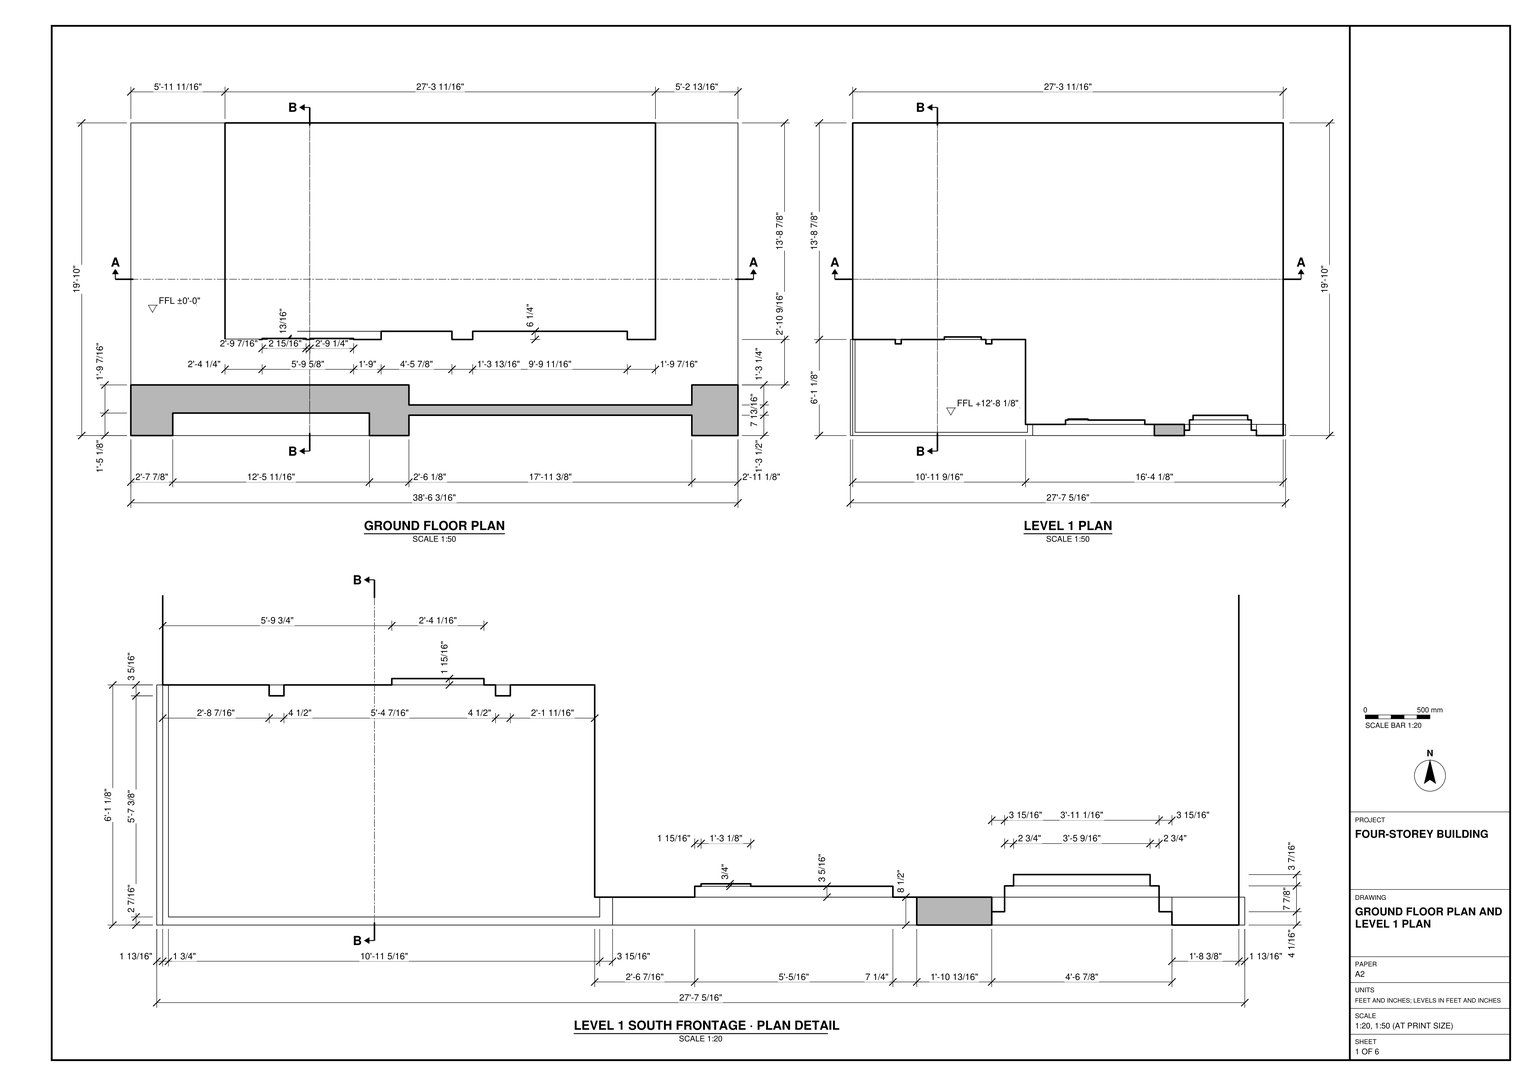
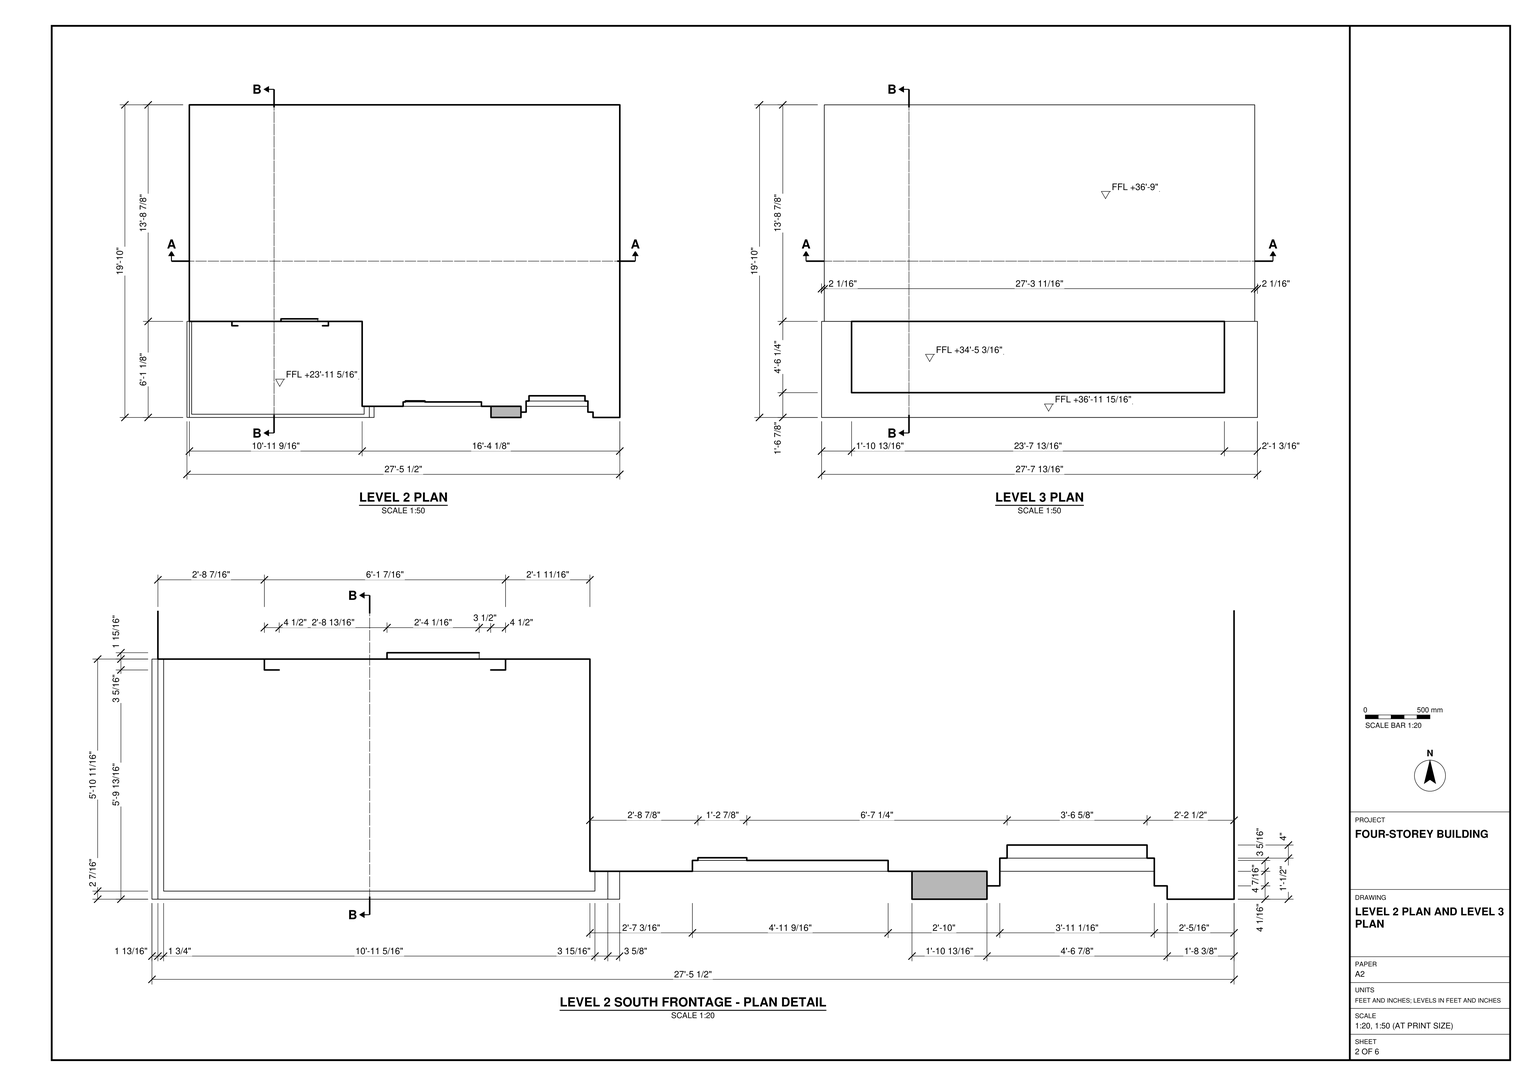
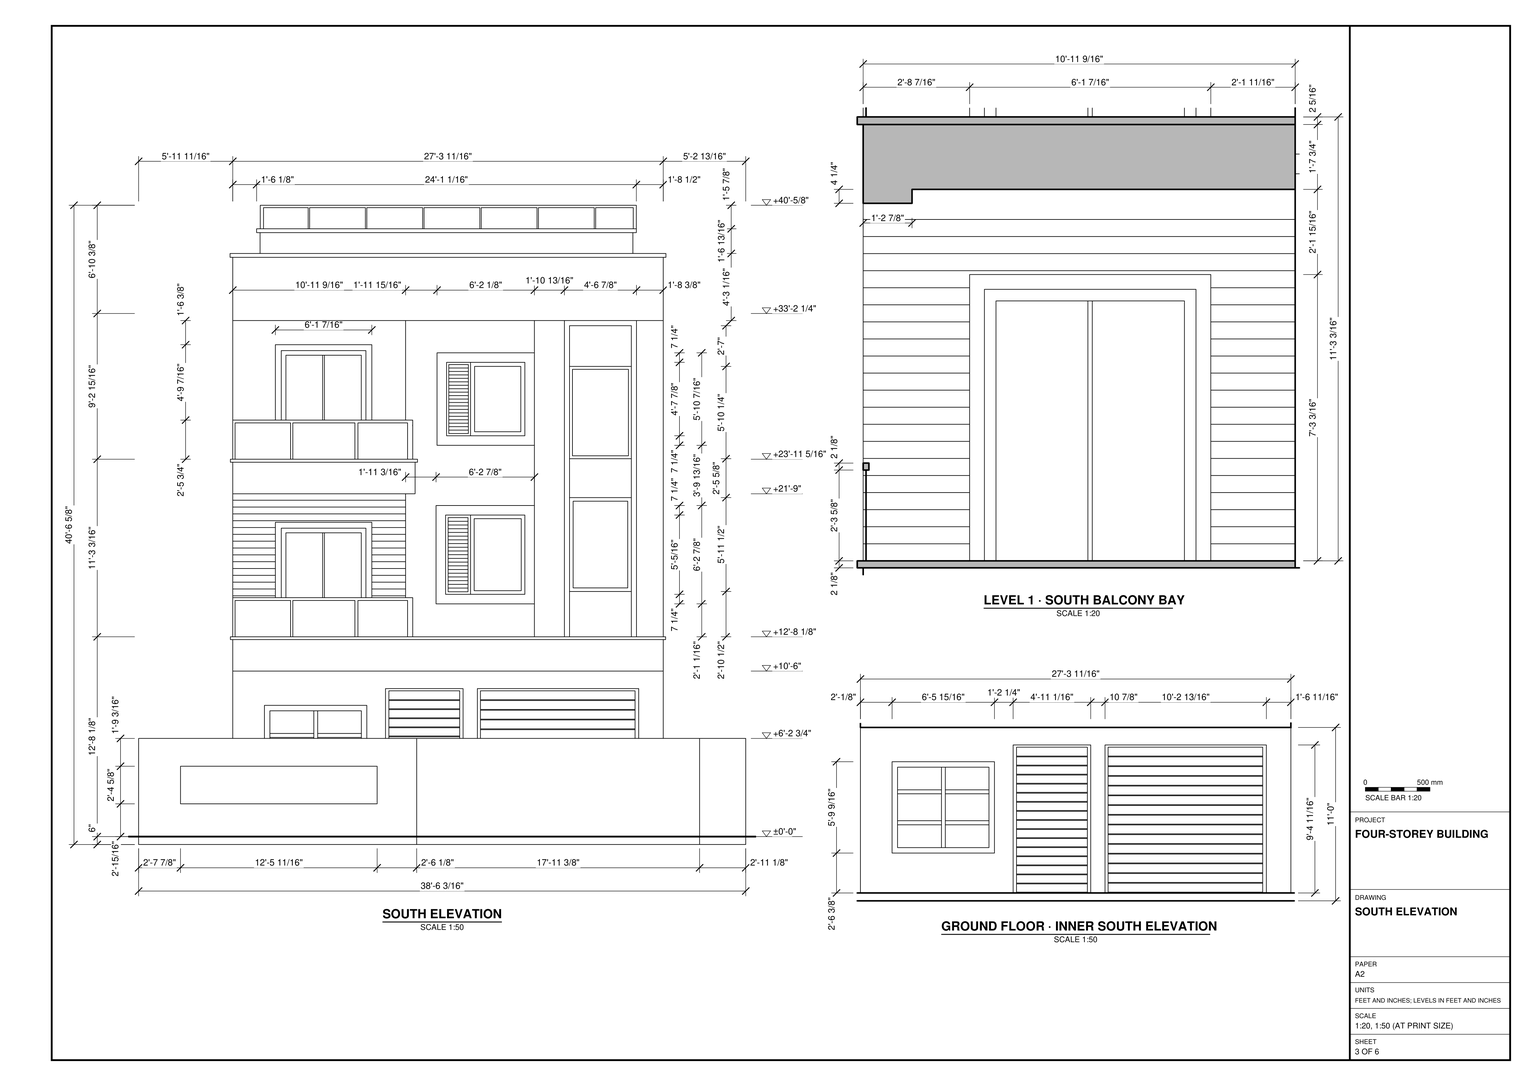
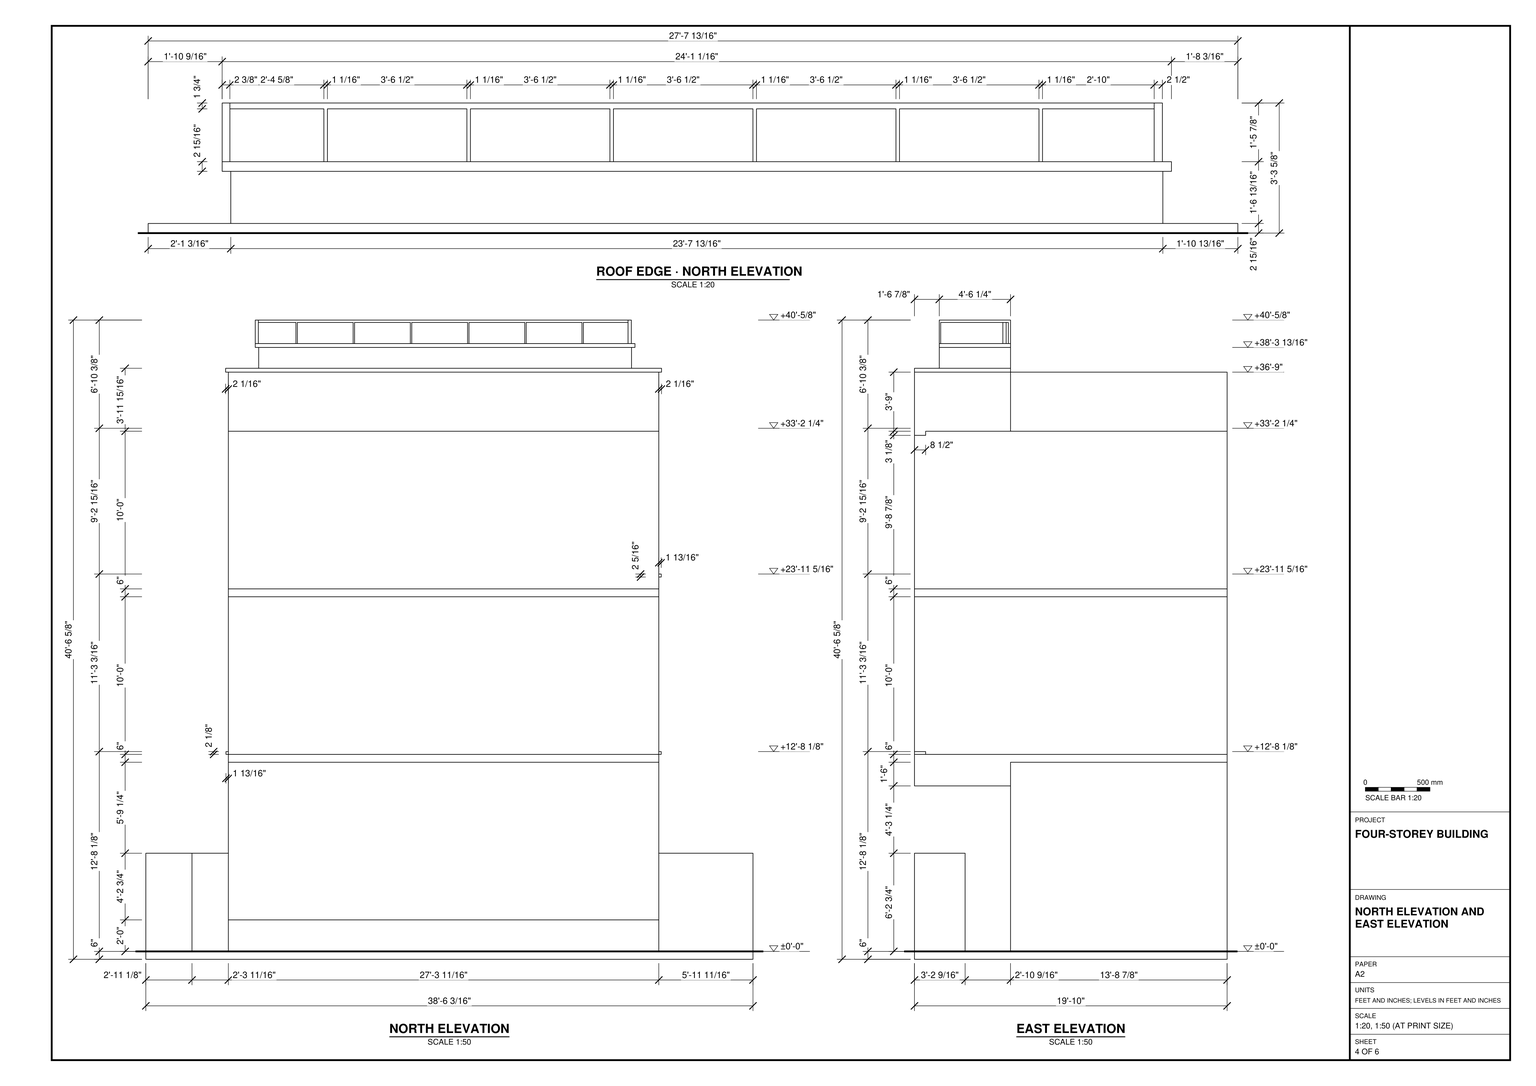
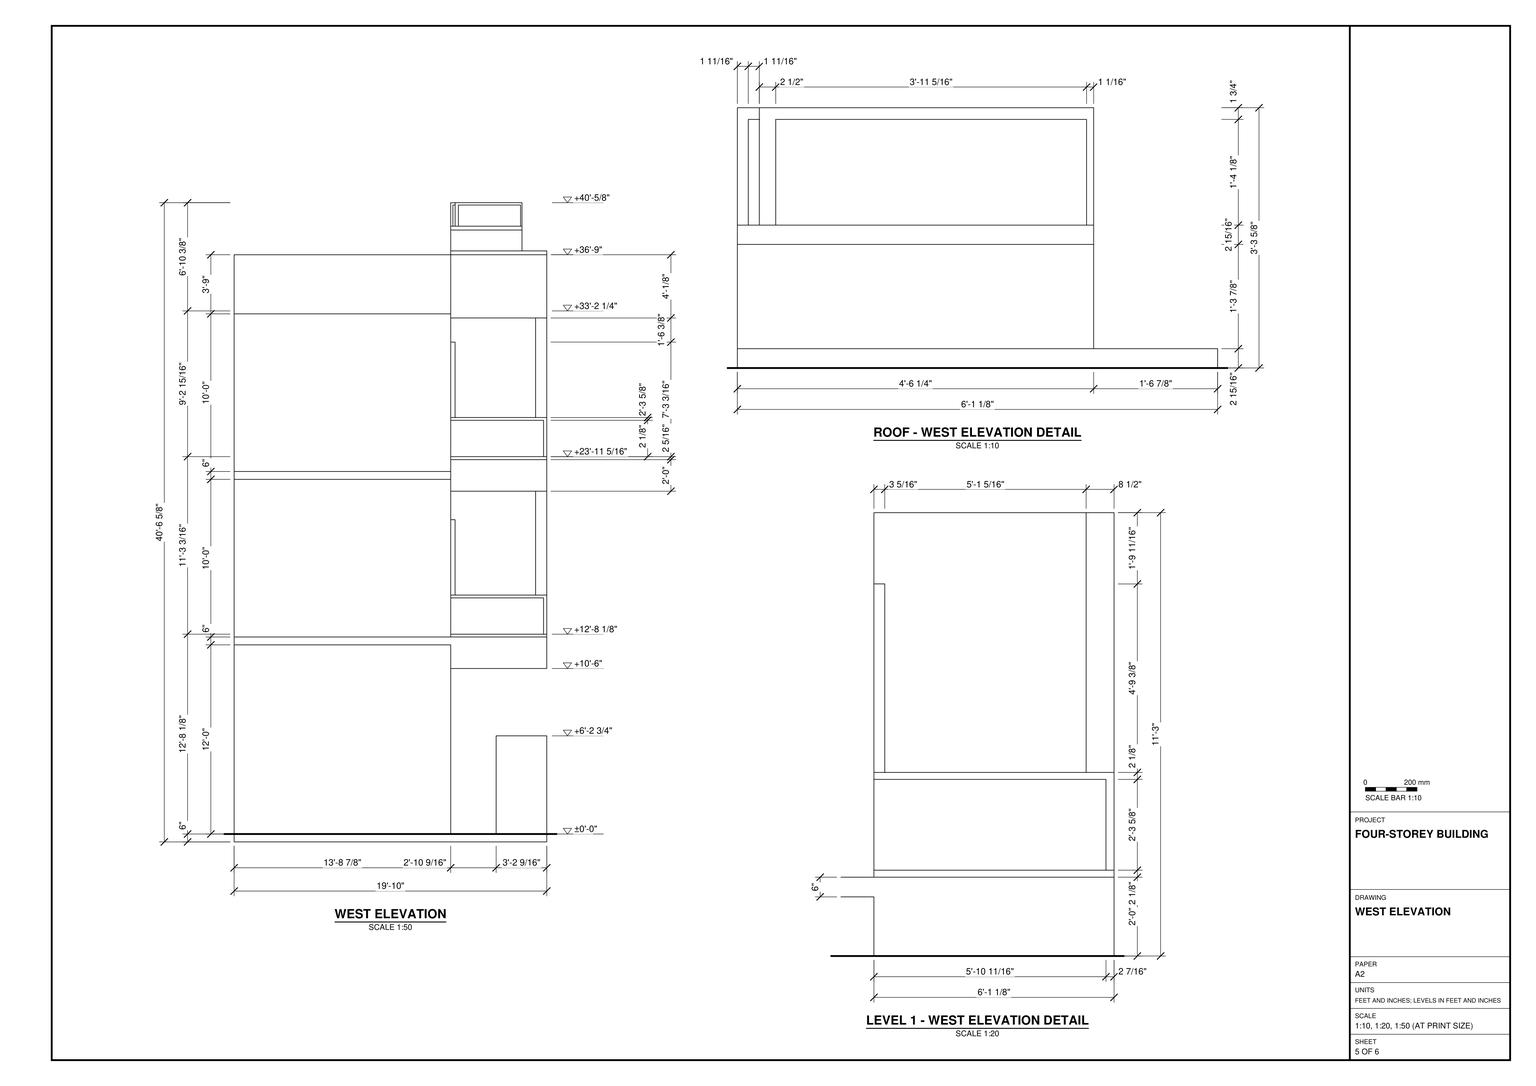
Build the four-storey building in SketchUp from task_files/diagram_01.pdf. Work in feet and inches. Set the overall width to 38'-6 3/16", depth to 19'-10" and height to 40'-6 5/8". Use ±0'-0" for the ground floor and +12'-8 1/8", +23'-11 5/16" and +33'-2 1/4" for the successive levels.

Set out the south frontage wall separately from the narrower building behind it. Match the wall thicknesses, setbacks and changes in profile to the plans. On the inner ground-floor elevation, place the divided window on the left and the narrow and wide horizontally slatted openings to its right. Model the floor slabs and stack the balconies on the left of the south elevation. Show their projecting slab edges, panelled guards and recessed paired doors. Use the enlarged balcony view for the horizontal courses around the lower balcony doors. To the right of the balconies, distinguish the windows with louvred side panels from the tall framed bay. Finish the roof with the changes in height shown in the level 3 plan and south elevation.

Keep shell elements such as walls, slabs and roof in separate groups or components. Keep each furniture or joinery piece shown separate and use components for repeated parts. Any decor or loose items shown may use suitable library components. Save one SketchUp model as output_files/four_storey_building_with_stacked_south_balconies.skp.

# SketchUp Ruby script. Lengths in inches.
U = 1.inch
M = Sketchup.active_model
def pt(a) = Geom::Point3d.new(a.map { |v| v * U })
def face(e, loops, mat)
  f = e.add_face(loops[0].map { |a| pt(a) })
  loops[1..].each { |l| e.add_face(l.map { |a| pt(a) }).erase! }
  f.material = f.back_material = mat if mat
  f
end
# faces: each face lists its corners as indices into pts; further lists are holes
def faces(e, pts, list, mat = nil) = list.each { |f| face(e, (f[0].is_a?(Array) ? f : [f]).map { |l| l.map { |i| pts[i] } }, mat) }
# xy, xz, yz: faces in a plane at the given z, y or x. An outline is a flat list of corners, or four numbers for a rectangle; further outlines are holes
def ring(l) = l.size == 4 ? [[l[0], l[1]], [l[2], l[1]], [l[2], l[3]], [l[0], l[3]]] : l.each_slice(2).to_a
def flat(e, list, mat, &to3) = list.each { |f| face(e, (f[0].is_a?(Array) ? f : [f]).map { |l| ring(l).map { |u, v| to3.(u, v) } }, mat) }
def xy(e, z, list, mat = nil) = flat(e, list, mat) { |x, y| [x, y, z] }
def xz(e, y, list, mat = nil) = flat(e, list, mat) { |x, z| [x, y, z] }
def yz(e, x, list, mat = nil) = flat(e, list, mat) { |y, z| [x, y, z] }
def lines(e, pts, list) = list.each { |a, b| e.add_line(pt(pts[a]), pt(pts[b])) }
# prism: a flat outline (further loops are holes) pulled along v
def prism(e, loops, v, mat = nil)
  f = face(e, loops, mat); d = Geom::Vector3d.new(v.map { |x| x * U })
  f.pushpull(f.normal.samedirection?(d) ? d.length : -d.length)
end
def box(e, o, s, mat = nil) = prism(e, [[o, [o[0] + s[0], o[1], o[2]], [o[0] + s[0], o[1] + s[1], o[2]], [o[0], o[1] + s[1], o[2]]]], [0, 0, s[2]], mat)
def at(x, y, z, deg = 0) = Geom::Transformation.translation(pt([x, y, z])) * Geom::Transformation.rotation(ORIGIN, Z_AXIS, deg.degrees)
def axes(o, x, y, z) = Geom::Transformation.new([*x, 0, *y, 0, *z, 0, *pt(o).to_a, 1])
def part(name) = M.definitions.add(name)
# library, detail: a bought-in or finely detailed component or shape, given as its bounding box
def library(name, o, s) = part(name).tap { |d| box(d.entities, o, s) }
def detail(e, o, s) = box(e.add_group.entities, o, s)
def put(e, d, t, mat = nil) = e.add_instance(d, t).tap { |i| i.material = mat if mat }
def group(e, t, mat = nil) = e.add_group.tap { |g| g.transformation = t; g.material = mat if mat }.entities
root = M.entities
M.materials.add("[0009_Linen]").color = [250, 240, 230]
M.materials.add("[0137_Black]").color = [0, 0, 0]
M.materials.add("[Translucent Glass Gray]").color = [252, 252, 252]
M.materials["[Translucent Glass Gray]"].alpha = 0.5
M.materials.add("[Wood Bamboo]").color = [177, 105, 43]
M.materials.add("[Wood Fence with Lattice]").color = [170, 106, 61]
xy(root,-24,[[0,0,0,238,462.1875,238,462.1875,0,427.0625,0,427.0625,15.5,211.7,15.5,211.7,0]])
xy(root,-18,[[211.7,23.29,427.0625,23.29,427.0625,38.54,462.1875,38.54,462.1875,238,399.375,238,399.375,73.125,377.92,73.125,377.92,79.375,260.24,79.375,260.24,73.125,244.4375,73.125,244.4375,79.375,190.53,79.375,190.53,73.125,71.6875,73.125,71.6875,238,0,238,0,38.54,211.7,38.54]])
xy(root,6.95,[[31.9,0,181.59,17.125]])
xy(root,16.52,[[99.95,73.125,133.38,73.9375],[136.32,73.125,169.5625,73.9375]])
xy(root,33.9,[[99.95,73.125,133.38,73.9375],[136.32,73.125,169.5625,73.9375]])
xy(root,35.58,[[31.9,0,181.59,17.125]])
xy(root,37.01,[[99.95,73.125,133.38,73.9375],[136.32,73.125,169.5625,73.9375]])
xy(root,56.75,[[0,0,211.7,38.54],[427.0625,0,462.1875,38.54],[211.7,15.5,427.0625,23.29]])
xy(root,57.5,[[99.95,73.125,133.38,73.9375],[136.32,73.125,169.5625,73.9375]])
xy(root,60.52,[[99.95,73.125,133.38,73.9375],[136.32,73.125,169.5625,73.9375]])
xy(root,77.76,[[99.95,73.125,133.38,73.9375],[136.32,73.125,169.5625,73.9375]])
xy(root,93,[[190.53,73.125,244.4375,79.375],[260.24,73.125,377.92,79.375]])
xy(root,108,[[71.6875,0,399.375,73.125]])
xy(root,126,[[71.6875,73.125,399.375,238]])
xy(root,132,[[69.875,0,71.6875,73.125],[71.6875,0,71.6875,73.125,203.24,73.125,203.24,8.5,399.375,8.5,399.375,0],[399.375,0,401.1875,8.5],[203.24,8.5,203.24,73.125,71.6875,73.125,71.6875,238,399.375,238,399.375,8.5]])
xy(root,134.125,[[69.875,0,71.6875,0,71.6875,2.46,72.5625,2.46,72.5625,73.125,69.875,73.125],[115.68,0,117.4,1.23],[164.67,0,166.96,1.23],[208.6875,0,301.31,0,301.31,8.5,206.72,8.5,206.72,2.46,208.6875,2.46],[301.31,0,324.14,8.5],
  [324.14,0,379.01,0,379.01,4.0625,375.09,4.0625,375.09,8.5,328.05,8.5,328.05,4.0625,324.14,4.0625],[379.01,0,399.375,8.5],[399.375,0,401.1875,8.5],[73.4375,1.23,115.68,1.23,115.68,2.46,117.4,2.46,117.4,1.23,164.67,1.23,164.67,2.46,166.96,2.46,166.96,1.23,204.76,1.23,204.76,2.46,206.72,2.46,206.72,8.5,203.24,8.5,203.24,73.125,177.54,73.125,177.54,69.8125,173.04,69.8125,173.04,73.125,108.61,73.125,108.61,69.8125,104.11,69.8125,104.11,73.125,72.5625,73.125,72.5625,2.46,73.4375,2.46],[115.68,1.23,117.4,2.46],
  [164.67,1.23,166.96,2.46],[324.14,4.0625,328.05,8.5],[375.09,4.0625,379.01,8.5],[104.11,69.8125,108.61,73.125],[173.04,69.8125,177.54,73.125],
  [141.45,73.125,169.52,75.0625]])
xy(root,134.125,[[73.4375,0,115.68,1.23],[117.4,0,164.67,1.23],[166.96,0,204.76,1.23]],"[0137_Black]")
xy(root,161.78,[[73.4375,0,115.68,1.23],[117.4,0,164.67,1.23],[166.96,0,204.76,1.23],[73.4375,1.23,115.68,2.46],[117.4,1.23,164.67,2.46],
  [166.96,1.23,204.76,2.46],[71.6875,2.46,72.5625,73.125],[72.5625,2.46,73.4375,73.125],[204.76,2.46,206.72,8.5],[206.72,2.46,208.6875,8.5]])
xy(root,163.9,[[71.6875,0,208.6875,0,208.6875,8.5,204.76,8.5,204.76,2.46,73.4375,2.46,73.4375,73.125,71.6875,73.125]],"[0137_Black]")
xy(root,166.46,[[233.7,8.5,294.04,11.8125]])
xy(root,168.39,[[235.63,11.8125,250.76,12.5625]])
xy(root,168.6,[[328.05,8.5,375.09,11.9375]])
xy(root,171.22,[[235.63,11.8125,250.76,12.5625]])
xy(root,171.34,[[330.79,11.9375,372.35,15.375]])
xy(root,174.04,[[235.63,11.8125,250.76,12.5625]])
xy(root,176.86,[[235.63,11.8125,250.76,12.5625]])
xy(root,179.6875,[[235.63,11.8125,250.76,12.5625]])
xy(root,182.51,[[235.63,11.8125,250.76,12.5625]])
xy(root,185.33,[[235.63,11.8125,250.76,12.5625]])
xy(root,188.16,[[235.63,11.8125,250.76,12.5625]])
xy(root,190.98,[[235.63,11.8125,250.76,12.5625]])
xy(root,193.8,[[235.63,11.8125,250.76,12.5625]])
xy(root,196.625,[[235.63,11.8125,250.76,12.5625]])
xy(root,199.45,[[235.63,11.8125,250.76,12.5625]])
xy(root,202.27,[[235.63,11.8125,250.76,12.5625]])
xy(root,205.1,[[235.63,11.8125,250.76,12.5625]])
xy(root,207.92,[[235.63,11.8125,250.76,12.5625]])
xy(root,210.74,[[235.63,11.8125,250.76,12.5625]])
xy(root,213.28,[[141.45,73.125,169.52,75.0625]])
xy(root,213.57,[[235.63,11.8125,250.76,12.5625]])
xy(root,216.39,[[235.63,11.8125,250.76,12.5625]])
xy(root,216.81,[[108.61,69.8125,173.04,73.125]])
xy(root,219.21,[[235.63,11.8125,250.76,12.5625]])
xy(root,221.3125,[[104.11,69.8125,177.54,73.125]])
xy(root,222.04,[[235.63,11.8125,250.76,12.5625]])
xy(root,226.8,[[233.7,8.5,294.04,11.8125]])
xy(root,237.36,[[330.79,11.9375,372.35,15.375]])
xy(root,240.1,[[328.05,8.5,375.09,11.9375]])
xy(root,243,[[71.6875,0,71.6875,73.125,86.57,73.125,86.57,8.5,210.49,8.5,210.49,0]])
xy(root,247.25,[[141.9,36.55,140.6,36.72,139.38,37.22,138.34,38.03,137.54,39.07,137.03,40.28,136.86,41.59,137.03,42.89,137.54,44.11,138.34,45.15,139.38,45.95,140.6,46.46,141.9,46.63,143.21,46.46,144.42,45.95,144.9,45.59,144.9,37.59,144.42,37.22,143.21,36.72],[144.9,37.59,144.9,45.59,145.47,45.15,146.27,44.11,146.77,42.89,146.94,41.59,146.77,40.28,146.27,39.07,145.47,38.03]])
xy(root,247.25,[[86.57,8.5,98.23,73.125],[98.23,8.5,109.9,73.125],[109.9,8.5,121.57,73.125],[121.57,8.5,133.24,73.125],[133.24,8.5,133.24,73.125,144.9,73.125,144.9,45.59,144.42,45.95,143.21,46.46,141.9,46.63,140.6,46.46,139.38,45.95,138.34,45.15,137.54,44.11,137.03,42.89,136.86,41.59,137.03,40.28,137.54,39.07,138.34,38.03,139.38,37.22,140.6,36.72,141.9,36.55,143.21,36.72,144.42,37.22,144.9,37.59,144.9,8.5],
  [144.9,8.5,144.9,37.59,145.47,38.03,146.27,39.07,146.77,40.28,146.94,41.59,146.77,42.89,146.27,44.11,145.47,45.15,144.9,45.59,144.9,73.125,156.57,73.125,156.57,8.5],[156.57,8.5,168.24,73.125],[168.24,8.5,179.9,73.125],[179.9,8.5,191.57,73.125],[191.57,8.5,203.24,73.125]],"[Wood Bamboo]")
xy(root,267,[[69.875,0,71.6875,73.125],[71.6875,0,71.6875,73.125,203.24,73.125,203.24,8.5,210.49,8.5,210.49,0],[210.49,0,212.3,8.5]])
xy(root,269.3125,[[71.6875,0,73.4375,2.46],[73.4375,0,208.6875,0,208.6875,2.46,206.72,2.46,206.72,8.5,203.24,8.5,203.24,73.125,72.5625,73.125,72.5625,2.46,73.4375,2.46],[208.6875,0,212.3,0,212.3,8.5,206.72,8.5,206.72,2.46,208.6875,2.46],[141.45,73.125,169.52,75.0625]])
xy(root,269.3125,[[69.875,0,71.6875,0,71.6875,2.46,72.5625,2.46,72.5625,73.125,69.875,73.125]],"[0137_Black]")
xy(root,269.7,[[328.05,8.5,375.09,12.5]])
xy(root,271.91,[[330.27,12.5,372.875,16.5]])
xy(root,287.15,[[234.45,8.5,294.04,11.8125]])
xy(root,288.84,[[236.13,11.8125,251.01,12.625]])
xy(root,291.46,[[236.13,11.8125,251.01,12.625]])
xy(root,294.09,[[236.13,11.8125,251.01,12.625]])
xy(root,296.72,[[236.13,11.8125,251.01,12.625]])
xy(root,296.97,[[73.4375,0,115.68,1.23],[73.4375,1.23,115.68,2.46],[166.96,1.23,204.76,2.46],[71.6875,2.46,72.5625,73.125],[72.5625,2.46,73.4375,73.125],
  [204.76,2.46,206.72,8.5],[206.72,2.46,208.6875,8.5]])
xy(root,299.09,[[71.6875,0,208.6875,0,208.6875,8.5,204.76,8.5,204.76,2.46,73.4375,2.46,73.4375,73.125,71.6875,73.125]],"[0137_Black]")
xy(root,299.34,[[236.13,11.8125,251.01,12.625]])
xy(root,301.97,[[236.13,11.8125,251.01,12.625]])
xy(root,304.6,[[236.13,11.8125,251.01,12.625]])
xy(root,307.22,[[236.13,11.8125,251.01,12.625]])
xy(root,309.85,[[236.13,11.8125,251.01,12.625]])
xy(root,312.48,[[236.13,11.8125,251.01,12.625]])
xy(root,315.1,[[236.13,11.8125,251.01,12.625]])
xy(root,317.73,[[236.13,11.8125,251.01,12.625]])
xy(root,320.36,[[236.13,11.8125,251.01,12.625]])
xy(root,322.98,[[236.13,11.8125,251.01,12.625]])
xy(root,325.61,[[236.13,11.8125,251.01,12.625]])
xy(root,328.24,[[236.13,11.8125,251.01,12.625]])
xy(root,330.86,[[236.13,11.8125,251.01,12.625]])
xy(root,333.49,[[236.13,11.8125,251.01,12.625]])
xy(root,336.12,[[236.13,11.8125,251.01,12.9375]])
xy(root,337.74,[[330.27,12.5,372.875,16.5]])
xy(root,338.74,[[236.13,11.8125,251.01,12.9375]])
xy(root,339.96,[[328.05,8.5,375.09,12.5]])
xy(root,343.05,[[234.45,8.5,294.04,11.8125]])
xy(root,356.5,[[104.11,69.8125,177.54,73.125]])
xy(root,370.96,[[328.05,4.0625,375.09,8.5]])
xy(root,374.875,[[71.6875,0,71.6875,73.125,87.05,73.125,87.05,8.5,301.31,8.5,301.31,0],[301.31,0,324.14,8.5],[324.14,0,379.01,4.0625],[379.01,0,399.375,8.5],[324.14,4.0625,379.01,8.5]])
xy(root,378,[[203.24,8.5,399.375,73.125],[106.19,32.41,104.73,32.6,103.38,33.16,102.21,34.06,101.32,35.22,100.76,36.58,100.57,38.03,100.76,39.49,101.32,40.85,102.21,42.01,103.38,42.91,104.73,43.47,106.19,43.66,107.65,43.47,109,42.91,110.17,42.01,110.29,41.86,111.0625,40.85,111.625,39.49,111.82,38.03,111.625,36.58,111.0625,35.22,110.29,34.21,110.17,34.06,109,33.16,107.65,32.6],[146.94,32.78,145.58,32.96,145.14,33.15,144.32,33.49,143.23,34.32,142.4,35.41,141.87,36.68,141.69,38.03,141.87,39.39,142.4,40.66,143.23,41.75,144.32,42.58,145.14,42.92,145.58,43.11,146.94,43.28,148.3,43.11,149.57,42.58,150.65,41.75,151.49,40.66,152.01,39.39,152.19,38.03,152.01,36.68,151.49,35.41,150.65,34.32,149.57,33.49,148.3,32.96],[71.6875,73.125,399.375,238]])
xy(root,378,[[87.05,8.5,98.67,73.125],[98.67,8.5,98.67,73.125,110.29,73.125,110.29,41.86,110.17,42.01,109,42.91,107.65,43.47,106.19,43.66,104.73,43.47,103.38,42.91,102.21,42.01,101.32,40.85,100.76,39.49,100.57,38.03,100.76,36.58,101.32,35.22,102.21,34.06,103.38,33.16,104.73,32.6,106.19,32.41,107.65,32.6,109,33.16,110.17,34.06,110.29,34.21,110.29,8.5],[110.29,8.5,110.29,34.21,111.0625,35.22,111.625,36.58,111.82,38.03,111.625,39.49,111.0625,40.85,110.29,41.86,110.29,73.125,121.9,73.125,121.9,8.5],[121.9,8.5,133.52,73.125],[133.52,8.5,133.52,73.125,145.14,73.125,145.14,42.92,144.32,42.58,143.23,41.75,142.4,40.66,141.87,39.39,141.69,38.03,141.87,36.68,142.4,35.41,143.23,34.32,144.32,33.49,145.14,33.15,145.14,8.5],
  [145.14,8.5,145.14,33.15,145.58,32.96,146.94,32.78,148.3,32.96,149.57,33.49,150.65,34.32,151.49,35.41,152.01,36.68,152.19,38.03,152.01,39.39,151.49,40.66,150.65,41.75,149.57,42.58,148.3,43.11,146.94,43.28,145.58,43.11,145.14,42.92,145.14,73.125,156.76,73.125,156.76,8.5],[156.76,8.5,168.38,73.125],[168.38,8.5,180,73.125],[180,8.5,191.62,73.125],[191.62,8.5,203.24,73.125]],"[Wood Bamboo]")
xy(root,380.25,[[87.05,8.5,203.24,73.125]])
xy(root,395.1875,[[87.05,8.5,203.24,73.125]])
xy(root,423,[[69.625,0,71.6875,73.125],[71.6875,0,399.375,73.125],[399.375,0,401.4375,73.125],[71.6875,73.125,399.375,238]])
xy(root,425.9375,[[69.625,0,401.4375,0,401.4375,73.125,376.28,73.125,376.28,18.875,92.46,18.875,92.46,73.125,69.625,73.125],[92.46,18.875,376.28,73.125]])
xy(root,441.8125,[[89.84,18.875,92.46,73.125],[92.46,18.875,376.28,73.125],[376.28,18.875,378.9,73.125]])
xy(root,444.75,[[[89.84,18.875,92.61,18.875,92.61,19.95,95.11,19.95,95.11,18.875,129.1,18.875,129.1,19.95,130.18,19.95,130.18,18.875,172.65,18.875,172.65,19.95,173.73,19.95,173.73,18.875,216.2,18.875,216.2,19.95,217.28,19.95,217.28,18.875,259.75,18.875,259.75,19.95,260.83,19.95,260.83,18.875,303.3,18.875,303.3,19.95,304.38,19.95,304.38,18.875,346.85,18.875,346.85,19.95,347.93,19.95,347.93,18.875,376.55,18.875,376.55,19.95,378.9,19.95,378.9,71.46,376.55,71.46,376.55,73.125,89.84,73.125],[92.61,67.28,95.11,69.78]],[92.61,67.28,95.11,69.78]])
xy(root,460.85,[[95.11,18.875,129.1,19.95],[130.18,18.875,172.65,19.95],[173.73,18.875,216.2,19.95],[217.28,18.875,259.75,19.95],[260.83,18.875,303.3,19.95],
  [304.38,18.875,346.85,19.95],[347.93,18.875,376.55,19.95],[92.61,19.95,95.11,67.28],[376.55,19.95,378.9,71.46]])
xy(root,462.625,[[92.61,18.875,378.9,18.875,378.9,73.125,376.55,73.125,376.55,19.95,95.11,19.95,95.11,69.78,92.61,69.78]])
xz(root,0,[[[0,-24,211.7,56.75],[31.9,6.95,181.59,35.58]],[427.0625,-24,462.1875,56.75]])
xz(root,0,[[71.6875,108,399.375,132],[301.31,134.125,324.14,374.875],[379.01,134.125,399.375,374.875],[71.6875,243,210.49,267],[71.6875,374.875,399.375,423]],"[0009_Linen]")
xz(root,0,[[69.875,132,401.1875,134.125],[71.6875,134.125,73.4375,134.125,73.4375,161.78,115.68,161.78,115.68,134.125,117.4,134.125,117.4,161.78,164.67,161.78,164.67,134.125,166.96,134.125,166.96,161.78,204.76,161.78,204.76,134.125,208.6875,134.125,208.6875,163.9,71.6875,163.9],[69.875,267,212.3,269.3125],[71.6875,269.3125,73.4375,269.3125,73.4375,296.97,115.68,296.97,115.68,269.3125,117.4,269.3125,117.4,296.97,164.67,296.97,164.67,269.3125,166.96,269.3125,166.96,296.97,204.76,296.97,204.76,269.3125,208.6875,269.3125,208.6875,299.09,71.6875,299.09],[69.625,423,401.4375,425.9375]],"[0137_Black]")
xz(root,0,[[166.96,269.3125,204.76,296.97]],"[Translucent Glass Gray]")
xz(root,1.23,[[166.96,269.3125,204.76,296.97]])
xz(root,1.23,[[73.4375,134.125,115.68,161.78],[117.4,134.125,164.67,161.78],[166.96,134.125,204.76,161.78],[73.4375,269.3125,115.68,296.97],[117.4,269.3125,164.67,296.97]],"[Translucent Glass Gray]")
xz(root,2.46,[[71.6875,134.125,72.5625,161.78],[72.5625,134.125,73.4375,161.78],[206.72,134.125,208.6875,161.78],[71.6875,269.3125,72.5625,296.97],[72.5625,269.3125,73.4375,296.97],
  [115.68,269.3125,115.68,296.97,73.4375,296.97,73.4375,299.09,204.76,299.09,204.76,296.97,166.96,296.97,166.96,269.3125,164.67,269.3125,164.67,296.97,117.4,296.97,117.4,269.3125],[204.76,269.3125,204.76,296.97,208.6875,296.97,208.6875,296.28,206.72,269.3125],[206.72,269.3125,208.6875,296.28,208.6875,269.3125]])
xz(root,2.46,[[115.68,134.125,115.68,161.78,73.4375,161.78,73.4375,163.9,204.76,163.9,204.76,161.78,166.96,161.78,166.96,134.125,164.67,134.125,164.67,161.78,117.4,161.78,117.4,134.125],[204.76,134.125,206.72,161.78]],"[0137_Black]")
xz(root,4.0625,[[324.14,134.125,328.05,134.125,328.05,370.96,375.09,370.96,375.09,134.125,379.01,134.125,379.01,374.875,324.14,374.875]])
xz(root,8.5,[[203.24,132,399.375,134.125],[399.375,132,401.1875,134.125],[301.31,134.125,324.14,374.875],[[226.43,159.1875,301.31,234.0625],[233.7,166.46,294.04,226.8]],[86.57,243,203.24,247.25],
  [203.24,243,210.49,252],[203.24,252,210.49,258],[203.24,258,210.49,267],[203.24,267,212.3,269.3125],[[227.18,279.88,301.31,350.32],[234.45,287.15,294.04,343.05]],
  [204.76,296.97,208.6875,299.09],[87.05,374.875,203.24,378],[203.24,374.875,324.14,378],[324.14,374.875,399.375,378],[87.05,378,203.24,380.25],
  [87.05,380.25,203.24,395.1875]])
xz(root,8.5,[[203.24,134.125,206.72,134.125,206.72,161.78,204.76,161.78,204.76,163.9,208.6875,163.9,208.6875,161.78,206.72,161.78,206.72,134.125,301.31,134.125,301.31,159.1875,226.43,159.1875,226.43,234.0625,301.31,234.0625,301.31,279.88,227.18,279.88,227.18,350.32,301.31,350.32,301.31,374.875,203.24,374.875,203.24,269.3125,206.72,269.3125,206.72,296.97,204.76,296.97,204.76,299.09,208.6875,299.09,208.6875,296.97,206.72,296.97,206.72,269.3125,212.3,269.3125,212.3,267,210.49,267,210.49,243,203.24,243],[328.05,134.125,375.09,168.6],[328.05,240.1,375.09,269.7],[328.05,339.96,375.09,370.96]],"[0009_Linen]")
xz(root,11.8125,[[[233.7,166.46,252.69,226.8],[235.63,168.39,250.76,224.86]],[[252.69,166.46,294.04,226.8],[255.45,169.21,291.28,224.04]],[[234.45,287.15,252.69,343.05],[236.13,288.84,251.01,341.37]],[[252.69,287.15,294.04,343.05],[255.77,290.23,290.96,339.97]]],"[0137_Black]")
xz(root,11.8125,[[255.45,169.21,291.28,224.04],[255.77,290.23,290.96,339.97]],"[Translucent Glass Gray]")
xz(root,11.8125,[[235.63,171.22,250.76,174.04],[235.63,176.86,250.76,179.6875],[235.63,182.51,250.76,185.33],[235.63,188.16,250.76,190.98],[235.63,193.8,250.76,196.625],
  [235.63,199.45,250.76,202.27],[235.63,205.1,250.76,207.92],[235.63,210.74,250.76,213.57],[235.63,216.39,250.76,219.21],[235.63,222.04,250.76,224.86],
  [236.13,291.46,251.01,294.09],[236.13,296.72,251.01,299.34],[236.13,301.97,251.01,304.6],[236.13,307.22,251.01,309.85],[236.13,312.48,251.01,315.1],
  [236.13,317.73,251.01,320.36],[236.13,322.98,251.01,325.61],[236.13,328.24,251.01,330.86],[236.13,333.49,251.01,336.12],[236.13,338.74,251.01,341.37]],"[Wood Bamboo]")
xz(root,11.9375,[[[328.05,168.6,375.09,240.1],[330.79,171.34,372.35,237.36]]],"[0137_Black]")
xz(root,12.5,[[[328.05,269.7,375.09,339.96],[330.27,271.91,372.875,337.74]]],"[0137_Black]")
xz(root,12.5625,[[235.63,168.39,250.76,171.22],[235.63,174.04,250.76,176.86],[235.63,179.6875,250.76,182.51],[235.63,185.33,250.76,188.16],[235.63,190.98,250.76,193.8],
  [235.63,196.625,250.76,199.45],[235.63,202.27,250.76,205.1],[235.63,207.92,250.76,210.74],[235.63,213.57,250.76,216.39],[235.63,219.21,250.76,222.04]])
xz(root,12.625,[[236.13,288.84,251.01,291.46],[236.13,294.09,251.01,296.72],[236.13,299.34,251.01,301.97],[236.13,304.6,251.01,307.22],[236.13,309.85,251.01,312.48],
  [236.13,315.1,251.01,317.73],[236.13,320.36,251.01,322.98],[236.13,325.61,251.01,328.24],[236.13,330.86,251.01,333.49]])
xz(root,12.9375,[[236.13,336.12,251.01,338.74]])
xz(root,15.375,[[330.79,171.34,372.35,237.36]],"[Translucent Glass Gray]")
xz(root,15.5,[[211.7,-24,427.0625,56.75]],"[Wood Fence with Lattice]")
xz(root,16.5,[[330.27,271.91,372.875,337.74]],"[Translucent Glass Gray]")
xz(root,17.125,[[31.9,6.95,181.59,35.58]])
xz(root,18.875,[[92.61,444.75,95.11,444.75,95.11,460.85,129.1,460.85,129.1,444.75,130.18,444.75,130.18,460.85,172.65,460.85,172.65,444.75,173.73,444.75,173.73,460.85,216.2,460.85,216.2,444.75,217.28,444.75,217.28,460.85,259.75,460.85,259.75,444.75,260.83,444.75,260.83,460.85,303.3,460.85,303.3,444.75,304.38,444.75,304.38,460.85,346.85,460.85,346.85,444.75,347.93,444.75,347.93,460.85,376.55,460.85,376.55,444.75,378.9,444.75,378.9,462.625,92.61,462.625]])
xz(root,18.875,[[92.46,425.9375,376.28,441.8125]],"[0009_Linen]")
xz(root,18.875,[[89.84,441.8125,378.9,444.75]],"[0137_Black]")
xz(root,19.95,[[92.61,444.75,95.11,460.85],[129.1,444.75,129.1,460.85,95.11,460.85,95.11,462.625,376.55,462.625,376.55,460.85,347.93,460.85,347.93,444.75,346.85,444.75,346.85,460.85,304.38,460.85,304.38,444.75,303.3,444.75,303.3,460.85,260.83,460.85,260.83,444.75,259.75,444.75,259.75,460.85,217.28,460.85,217.28,444.75,216.2,444.75,216.2,460.85,173.73,460.85,173.73,444.75,172.65,444.75,172.65,460.85,130.18,460.85,130.18,444.75],[376.55,444.75,378.9,460.85]])
xz(root,23.29,[[211.7,-18,427.0625,56.75]])
xz(root,38.54,[[0,-18,211.7,56.75],[427.0625,-18,462.1875,56.75]])
xz(root,67.28,[[92.61,444.75,95.11,460.85]])
xz(root,69.78,[[92.61,444.75,95.11,462.625]])
xz(root,69.8125,[[104.11,134.125,108.61,134.125,108.61,216.81,173.04,216.81,173.04,134.125,177.54,134.125,177.54,221.3125,104.11,221.3125],[104.11,269.3125,108.61,269.3125,108.61,352,173.04,352,173.04,269.3125,177.54,269.3125,177.54,356.5,104.11,356.5]])
xz(root,71.46,[[376.55,444.75,378.9,460.85]])
xz(root,73.125,[[[71.6875,-18,187.95,-18,187.95,94.6875,247.01,94.6875,247.01,-18,257.89,-18,257.89,94.6875,380.71,94.6875,380.71,-18,399.375,-18,399.375,108,71.6875,108],[95.79,12.36,173.72,81.92]],[187.95,-18,190.53,-18,190.53,93,244.4375,93,244.4375,-18,247.01,-18,247.01,94.6875,187.95,94.6875],[257.89,-18,260.24,-18,260.24,93,377.92,93,377.92,-18,380.71,-18,380.71,94.6875,257.89,94.6875],[[95.79,12.36,173.72,81.92],[99.95,16.52,169.5625,77.76]],[133.38,16.52,136.32,77.76],
  [99.95,33.9,133.38,37.01],[136.32,33.9,169.5625,37.01],[99.95,57.5,133.38,60.52],[136.32,57.5,169.5625,60.52],[71.6875,108,399.375,126],
  [69.875,132,71.6875,134.125],[71.6875,132,203.24,134.125],[71.6875,134.125,72.5625,139.32],[108.61,134.125,112.13,134.125,112.13,213.28,169.52,213.28,169.52,134.125,173.04,134.125,173.04,216.81,108.61,216.81],[112.13,134.125,140.12,213.28],
  [140.12,134.125,141.45,213.28],[71.6875,139.32,72.5625,144.52],[71.6875,144.52,72.5625,149.72],[71.6875,149.72,72.5625,154.92],[71.6875,154.92,72.5625,160.12],
  [71.6875,160.12,72.5625,161.78],[71.6875,161.78,73.4375,163.9],[71.6875,243,86.57,243,86.57,247.25,203.24,247.25,203.24,252,71.6875,252],[71.6875,252,203.24,258],[71.6875,258,203.24,267],
  [69.875,267,71.6875,269.3125],[71.6875,267,203.24,269.3125],[71.6875,269.3125,72.5625,296.97],[104.11,269.3125,108.61,269.3125,108.61,352,173.04,352,173.04,269.3125,177.54,269.3125,177.54,356.5,104.11,356.5],[108.61,269.3125,112.13,269.3125,112.13,348.47,169.52,348.47,169.52,269.3125,173.04,269.3125,173.04,352,108.61,352],
  [112.13,269.3125,140.12,348.47],[140.12,269.3125,141.45,348.47],[141.45,269.3125,169.52,348.47],[71.6875,296.97,73.4375,299.09],[71.6875,374.875,87.05,378],
  [71.6875,378,71.6875,423,399.375,423,399.375,378,203.24,378,203.24,395.1875,87.05,395.1875,87.05,378],[87.05,378,203.24,380.25],[87.05,380.25,203.24,395.1875],[69.625,423,401.4375,425.9375],[92.46,425.9375,376.28,441.8125],
  [89.84,441.8125,378.9,444.75],[376.55,444.75,378.9,462.625]])
xz(root,73.125,[[72.5625,269.3125,104.11,269.3125,104.11,356.5,177.54,356.5,177.54,269.3125,203.24,269.3125,203.24,378,87.05,378,87.05,374.875,71.6875,374.875,71.6875,299.09,73.4375,299.09,73.4375,296.97,72.5625,296.97]],"[0009_Linen]")
xz(root,73.125,[[72.5625,134.125,104.11,139.32],[177.54,134.125,203.24,139.32],[72.5625,139.32,104.11,144.52],[177.54,139.32,203.24,144.52],[72.5625,144.52,104.11,149.72],
  [177.54,144.52,203.24,149.72],[72.5625,149.72,104.11,154.92],[177.54,149.72,203.24,154.92],[72.5625,154.92,104.11,160.12],[177.54,154.92,203.24,160.12],
  [72.5625,160.12,104.11,160.12,104.11,165.3125,71.6875,165.3125,71.6875,163.9,73.4375,163.9,73.4375,161.78,72.5625,161.78],[177.54,160.12,203.24,165.3125],[71.6875,165.3125,104.11,170.51],[177.54,165.3125,203.24,170.51],[71.6875,170.51,104.11,175.71],
  [177.54,170.51,203.24,175.71],[71.6875,175.71,104.11,180.91],[177.54,175.71,203.24,180.91],[71.6875,180.91,104.11,186.11],[177.54,180.91,203.24,186.11],
  [71.6875,186.11,104.11,191.3],[177.54,186.11,203.24,191.3],[71.6875,191.3,104.11,196.5],[177.54,191.3,203.24,196.5],[71.6875,196.5,104.11,201.7],
  [177.54,196.5,203.24,201.7],[71.6875,201.7,104.11,206.9],[177.54,201.7,203.24,206.9],[71.6875,206.9,104.11,212.1],[177.54,206.9,203.24,212.1],
  [71.6875,212.1,104.11,217.29],[177.54,212.1,203.24,217.29],[71.6875,217.29,104.11,217.29,104.11,221.3125,177.54,221.3125,177.54,217.29,203.24,217.29,203.24,222.49,71.6875,222.49],[71.6875,222.49,203.24,227.69],[71.6875,227.69,203.24,232.89],
  [71.6875,232.89,203.24,238.09],[71.6875,238.09,203.24,238.09,203.24,247.25,86.57,247.25,86.57,243,71.6875,243]],"[Wood Bamboo]")
xz(root,73.9375,[[99.95,16.52,133.38,33.9],[136.32,16.52,169.5625,33.9],[99.95,37.01,133.38,57.5],[136.32,37.01,169.5625,57.5],[99.95,60.52,133.38,77.76],
  [136.32,60.52,169.5625,77.76]],"[Translucent Glass Gray]")
xz(root,75.0625,[[141.45,134.125,169.52,213.28],[141.45,269.3125,169.52,348.47]])
xz(root,79.375,[[190.53,-18,244.4375,-17.38],[260.24,-18,377.92,-17.38],[190.53,-11.09,244.4375,-10.48],[260.24,-10.6,377.92,-9.98],[190.53,-4.1875,244.4375,-3.57],
  [260.24,-3.2,377.92,-2.58],[190.53,2.72,244.4375,3.34],[260.24,4.2,377.92,4.82],[190.53,9.625,244.4375,10.24],[260.24,11.6,377.92,12.22],
  [190.53,16.53,244.4375,17.15],[260.24,19,377.92,19.62],[190.53,23.44,244.4375,24.06],[260.24,26.4,377.92,27.02],[190.53,30.35,244.4375,30.96],
  [260.24,33.8,377.92,34.42],[190.53,37.25,244.4375,37.87],[260.24,41.2,377.92,41.82],[190.53,44.16,244.4375,44.78],[260.24,48.6,377.92,49.22],
  [190.53,51.07,244.4375,51.68],[260.24,56,377.92,56.62],[190.53,57.97,244.4375,58.59],[260.24,63.4,377.92,64.02],[190.53,64.88,244.4375,65.5],
  [260.24,70.8,377.92,71.42],[190.53,71.79,244.4375,72.4],[260.24,78.2,377.92,78.82],[190.53,78.69,244.4375,79.31],[190.53,85.6,244.4375,86.22],
  [260.24,85.6,377.92,86.22]])
xz(root,79.375,[[190.53,-17.38,244.4375,-11.09],[260.24,-17.38,377.92,-10.6],[190.53,-10.48,244.4375,-4.1875],[260.24,-9.98,377.92,-3.2],[190.53,-3.57,244.4375,2.72],
  [260.24,-2.58,377.92,4.2],[190.53,3.34,244.4375,9.625],[260.24,4.82,377.92,11.6],[190.53,10.24,244.4375,16.53],[260.24,12.22,377.92,19],
  [190.53,17.15,244.4375,23.44],[260.24,19.62,377.92,26.4],[190.53,24.06,244.4375,30.35],[260.24,27.02,377.92,33.8],[190.53,30.96,244.4375,37.25],
  [260.24,34.42,377.92,41.2],[190.53,37.87,244.4375,44.16],[260.24,41.82,377.92,48.6],[190.53,44.78,244.4375,51.07],[260.24,49.22,377.92,56],
  [190.53,51.68,244.4375,57.97],[260.24,56.62,377.92,63.4],[190.53,58.59,244.4375,64.88],[260.24,64.02,377.92,70.8],[190.53,65.5,244.4375,71.79],
  [260.24,71.42,377.92,78.2],[190.53,72.4,244.4375,78.69],[260.24,78.82,377.92,85.6],[190.53,79.31,244.4375,85.6],[190.53,86.22,244.4375,93],
  [260.24,86.22,377.92,93]],"[Wood Bamboo]")
xz(root,238,[[0,-24,0,-18,71.6875,-18,71.6875,6,399.375,6,399.375,-18,462.1875,-18,462.1875,-24],[71.6875,6,399.375,126],[71.6875,126,399.375,132],[71.6875,132,399.375,252],[71.6875,252,399.375,258],
  [71.6875,258,399.375,378],[71.6875,378,399.375,423]])
yz(root,0,[[0,-24,0,56.75,38.54,56.75,38.54,-18,238,-18,238,-24]])
yz(root,31.9,[[0,6.95,17.125,35.58]])
yz(root,69.625,[[0,423,73.125,425.9375]],"[0137_Black]")
yz(root,69.875,[[0,132,73.125,134.125],[0,267,73.125,269.3125]],"[0137_Black]")
yz(root,71.6875,[[73.125,-18,238,126],[0,108,0,132,238,132,238,126,73.125,126,73.125,108],[73.125,132,238,252],[0,243,73.125,267],[73.125,252,238,258],
  [73.125,258,238,378],[0,374.875,73.125,423],[73.125,378,238,423]])
yz(root,71.6875,[[0,134.125,0,163.9,73.125,163.9,73.125,161.78,2.46,161.78,2.46,134.125],[0,269.3125,0,299.09,73.125,299.09,73.125,296.97,2.46,296.97,2.46,269.3125]],"[0137_Black]")
yz(root,72.5625,[[2.46,134.125,73.125,161.78],[2.46,269.3125,73.125,296.97]],"[Translucent Glass Gray]")
yz(root,73.4375,[[1.23,134.125,2.46,161.78],[0,269.3125,1.23,296.97],[1.23,269.3125,2.46,296.97],[2.46,296.97,73.125,299.09]])
yz(root,73.4375,[[0,134.125,1.23,161.78],[2.46,161.78,73.125,163.9]],"[0137_Black]")
yz(root,86.57,[[8.5,243,73.125,247.25]])
yz(root,87.05,[[8.5,374.875,73.125,378],[8.5,378,73.125,380.25],[8.5,380.25,73.125,395.1875]])
yz(root,89.84,[[18.875,441.8125,73.125,444.75]],"[0137_Black]")
yz(root,92.46,[[18.875,425.9375,73.125,441.8125]])
yz(root,92.61,[[18.875,444.75,18.875,462.625,69.78,462.625,69.78,444.75,67.28,444.75,67.28,460.85,19.95,460.85,19.95,444.75]])
yz(root,95.11,[[18.875,444.75,19.95,460.85],[67.28,444.75,69.78,444.75,69.78,462.625,19.95,462.625,19.95,460.85,67.28,460.85]])
yz(root,99.95,[[73.125,16.52,73.9375,33.9],[73.125,37.01,73.9375,57.5],[73.125,60.52,73.9375,77.76]])
yz(root,104.11,[[69.8125,134.125,73.125,221.3125],[69.8125,269.3125,73.125,356.5]])
yz(root,108.61,[[69.8125,134.125,73.125,216.81]])
yz(root,115.68,[[1.23,269.3125,2.46,296.97]])
yz(root,115.68,[[0,134.125,1.23,161.78],[1.23,134.125,2.46,161.78]],"[0137_Black]")
yz(root,117.4,[[1.23,134.125,2.46,161.78]])
yz(root,117.4,[[0,134.125,1.23,161.78]],"[0137_Black]")
yz(root,129.1,[[18.875,444.75,19.95,460.85]])
yz(root,130.18,[[18.875,444.75,19.95,460.85]])
yz(root,133.38,[[73.125,16.52,73.9375,33.9],[73.125,37.01,73.9375,57.5],[73.125,60.52,73.9375,77.76]])
yz(root,136.32,[[73.125,16.52,73.9375,33.9],[73.125,37.01,73.9375,57.5],[73.125,60.52,73.9375,77.76]])
yz(root,141.45,[[73.125,134.125,75.0625,213.28],[73.125,269.3125,75.0625,348.47]])
yz(root,164.67,[[1.23,269.3125,2.46,296.97]])
yz(root,164.67,[[0,134.125,1.23,161.78],[1.23,134.125,2.46,161.78]],"[0137_Black]")
yz(root,166.96,[[1.23,134.125,2.46,161.78]])
yz(root,166.96,[[0,134.125,1.23,161.78]],"[0137_Black]")
yz(root,169.52,[[73.125,134.125,75.0625,213.28]])
yz(root,169.5625,[[73.125,16.52,73.9375,33.9],[73.125,37.01,73.9375,57.5],[73.125,60.52,73.9375,77.76]])
yz(root,172.65,[[18.875,444.75,19.95,460.85]])
yz(root,173.04,[[69.8125,134.125,73.125,216.81]])
yz(root,173.73,[[18.875,444.75,19.95,460.85]])
yz(root,177.54,[[69.8125,134.125,73.125,221.3125],[69.8125,269.3125,73.125,356.5]])
yz(root,181.59,[[0,6.95,17.125,35.58]])
yz(root,190.53,[[73.125,-18,79.375,93]])
yz(root,203.24,[[8.5,132,73.125,134.125],[8.5,134.125,73.125,247.25],[8.5,247.25,73.125,252],[8.5,252,73.125,258],[8.5,258,73.125,267],
  [8.5,267,73.125,269.3125],[8.5,269.3125,73.125,378],[8.5,378,73.125,380.25],[8.5,380.25,73.125,395.1875]])
yz(root,204.76,[[1.23,269.3125,2.46,296.97],[2.46,296.97,8.5,299.09]])
yz(root,204.76,[[0,134.125,1.23,161.78],[1.23,134.125,2.46,161.78],[2.46,161.78,8.5,163.9]],"[0137_Black]")
yz(root,206.72,[[2.46,134.125,8.5,161.78]])
yz(root,208.6875,[[0,134.125,2.46,134.125,2.46,161.78,8.5,161.78,8.5,163.9,0,163.9],[0,269.3125,2.46,269.3125,2.46,296.97,8.5,296.97,8.5,299.09,0,299.09]],"[0137_Black]")
yz(root,210.49,[[0,243,8.5,267]])
yz(root,211.7,[[0,-24,15.5,56.75],[23.29,-18,38.54,56.75]])
yz(root,212.3,[[0,267,8.5,269.3125]],"[0137_Black]")
yz(root,216.2,[[18.875,444.75,19.95,460.85]])
yz(root,217.28,[[18.875,444.75,19.95,460.85]])
yz(root,233.7,[[8.5,166.46,11.8125,226.8]])
yz(root,234.45,[[8.5,287.15,11.8125,343.05]])
yz(root,235.63,[[11.8125,168.39,12.5625,171.22],[11.8125,174.04,12.5625,176.86],[11.8125,179.6875,12.5625,182.51],[11.8125,185.33,12.5625,188.16],[11.8125,190.98,12.5625,193.8],
  [11.8125,196.625,12.5625,199.45],[11.8125,202.27,12.5625,205.1],[11.8125,207.92,12.5625,210.74],[11.8125,213.57,12.5625,216.39],[11.8125,219.21,12.5625,222.04]])
yz(root,236.13,[[11.8125,288.84,12.625,291.46],[11.8125,294.09,12.625,296.72],[11.8125,299.34,12.625,301.97],[11.8125,304.6,12.625,307.22],[11.8125,309.85,12.625,312.48],
  [11.8125,315.1,12.625,317.73],[11.8125,320.36,12.625,322.98],[11.8125,325.61,12.625,328.24],[11.8125,330.86,12.625,333.49],[11.8125,336.12,12.9375,338.74]])
yz(root,244.4375,[[73.125,-18,79.375,93]])
yz(root,250.76,[[11.8125,168.39,12.5625,171.22],[11.8125,174.04,12.5625,176.86],[11.8125,179.6875,12.5625,182.51],[11.8125,185.33,12.5625,188.16],[11.8125,190.98,12.5625,193.8],
  [11.8125,196.625,12.5625,199.45],[11.8125,202.27,12.5625,205.1],[11.8125,207.92,12.5625,210.74],[11.8125,213.57,12.5625,216.39],[11.8125,219.21,12.5625,222.04]])
yz(root,251.01,[[11.8125,288.84,12.625,291.46],[11.8125,294.09,12.625,296.72],[11.8125,299.34,12.625,301.97],[11.8125,304.6,12.625,307.22],[11.8125,309.85,12.625,312.48],
  [11.8125,315.1,12.625,317.73],[11.8125,320.36,12.625,322.98],[11.8125,325.61,12.625,328.24],[11.8125,330.86,12.625,333.49],[11.8125,336.12,12.9375,338.74]])
yz(root,259.75,[[18.875,444.75,19.95,460.85]])
yz(root,260.24,[[73.125,-18,79.375,93]])
yz(root,260.83,[[18.875,444.75,19.95,460.85]])
yz(root,294.04,[[8.5,166.46,11.8125,226.8],[8.5,287.15,11.8125,343.05]])
yz(root,301.31,[[0,134.125,8.5,374.875]])
yz(root,303.3,[[18.875,444.75,19.95,460.85]])
yz(root,304.38,[[18.875,444.75,19.95,460.85]])
yz(root,324.14,[[0,134.125,4.0625,374.875],[4.0625,134.125,8.5,374.875]])
yz(root,328.05,[[4.0625,134.125,8.5,134.125,8.5,168.6,11.9375,168.6,11.9375,240.1,8.5,240.1,8.5,269.7,12.5,269.7,12.5,339.96,8.5,339.96,8.5,370.96,4.0625,370.96]])
yz(root,330.27,[[12.5,271.91,16.5,337.74]])
yz(root,330.79,[[11.9375,171.34,15.375,237.36]])
yz(root,346.85,[[18.875,444.75,19.95,460.85]])
yz(root,347.93,[[18.875,444.75,19.95,460.85]])
yz(root,372.35,[[11.9375,171.34,15.375,237.36]])
yz(root,372.875,[[12.5,271.91,16.5,337.74]])
yz(root,375.09,[[4.0625,134.125,4.0625,370.96,8.5,370.96,8.5,339.96,12.5,339.96,12.5,269.7,8.5,269.7,8.5,240.1,11.9375,240.1,11.9375,168.6,8.5,168.6,8.5,134.125]])
yz(root,376.28,[[18.875,425.9375,73.125,441.8125]])
yz(root,376.55,[[18.875,444.75,19.95,460.85],[71.46,444.75,71.46,460.85,19.95,460.85,19.95,462.625,73.125,462.625,73.125,444.75]])
yz(root,377.92,[[73.125,-18,79.375,93]])
yz(root,378.9,[[18.875,444.75,19.95,444.75,19.95,460.85,71.46,460.85,71.46,444.75,73.125,444.75,73.125,462.625,18.875,462.625]])
yz(root,378.9,[[18.875,441.8125,73.125,444.75]],"[0137_Black]")
yz(root,379.01,[[0,134.125,4.0625,374.875]])
yz(root,399.375,[[73.125,-18,238,126],[0,108,73.125,108,73.125,126,238,126,238,132,0,132],[8.5,132,238,132,238,252,0,252,0,134.125,8.5,134.125],[0,252,238,258],[0,258,238,258,238,378,8.5,378,8.5,374.875,0,374.875],
  [0,374.875,8.5,374.875,8.5,378,73.125,378,73.125,423,0,423],[73.125,378,238,423]])
yz(root,401.1875,[[0,132,8.5,134.125]])
yz(root,401.4375,[[0,423,73.125,425.9375]],"[0137_Black]")
yz(root,427.0625,[[0,-24,15.5,56.75],[23.29,-18,38.54,56.75]])
yz(root,462.1875,[[0,-24,238,-24,238,-18,38.54,-18,38.54,56.75,0,56.75]])
# 63 loose lines left out
